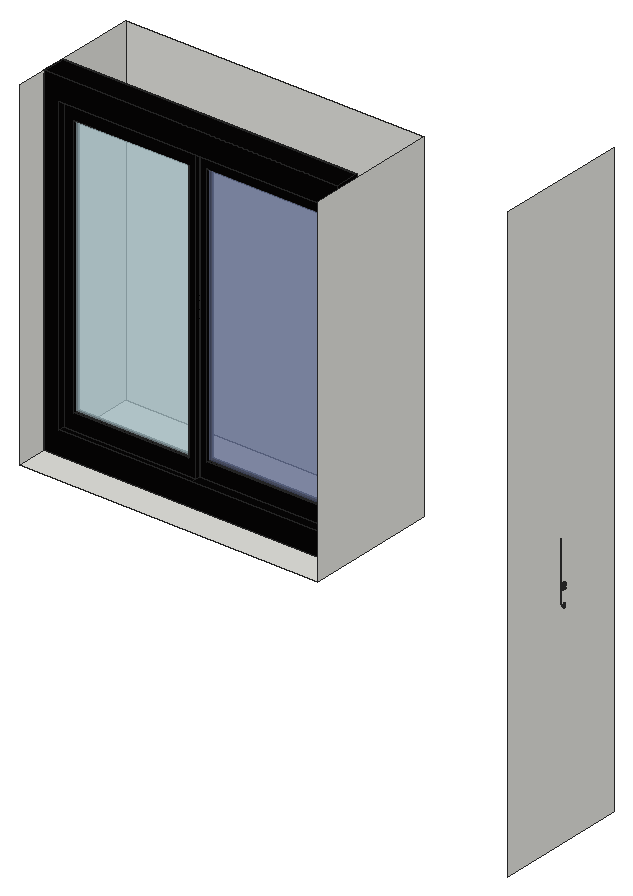
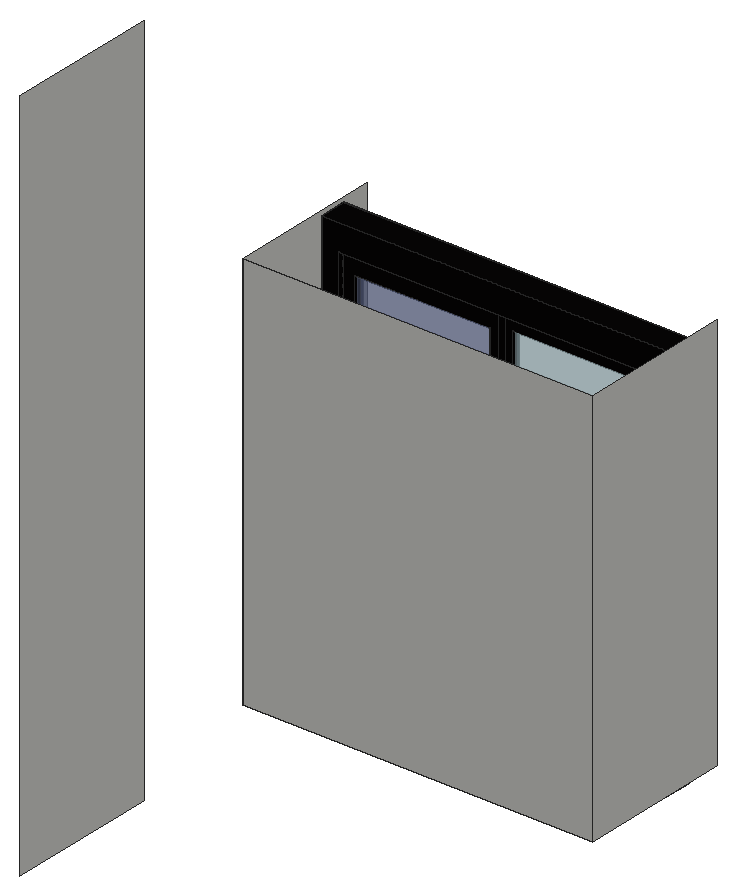
# SketchUp Ruby script. Lengths in inches.
U = 1.inch
M = Sketchup.active_model
def pt(a) = Geom::Point3d.new(a.map { |v| v * U })
def face(e, loops, mat)
  f = e.add_face(loops[0].map { |a| pt(a) })
  loops[1..].each { |l| e.add_face(l.map { |a| pt(a) }).erase! }
  f.material = f.back_material = mat if mat
  f
end
# faces: each face lists its corners as indices into pts; further lists are holes
def faces(e, pts, list, mat = nil) = list.each { |f| face(e, (f[0].is_a?(Array) ? f : [f]).map { |l| l.map { |i| pts[i] } }, mat) }
# xy, xz, yz: faces in a plane at the given z, y or x. An outline is a flat list of corners, or four numbers for a rectangle; further outlines are holes
def ring(l) = l.size == 4 ? [[l[0], l[1]], [l[2], l[1]], [l[2], l[3]], [l[0], l[3]]] : l.each_slice(2).to_a
def flat(e, list, mat, &to3) = list.each { |f| face(e, (f[0].is_a?(Array) ? f : [f]).map { |l| ring(l).map { |u, v| to3.(u, v) } }, mat) }
def xy(e, z, list, mat = nil) = flat(e, list, mat) { |x, y| [x, y, z] }
def xz(e, y, list, mat = nil) = flat(e, list, mat) { |x, z| [x, y, z] }
def yz(e, x, list, mat = nil) = flat(e, list, mat) { |y, z| [x, y, z] }
def lines(e, pts, list) = list.each { |a, b| e.add_line(pt(pts[a]), pt(pts[b])) }
# prism: a flat outline (further loops are holes) pulled along v
def prism(e, loops, v, mat = nil)
  f = face(e, loops, mat); d = Geom::Vector3d.new(v.map { |x| x * U })
  f.pushpull(f.normal.samedirection?(d) ? d.length : -d.length)
end
def box(e, o, s, mat = nil) = prism(e, [[o, [o[0] + s[0], o[1], o[2]], [o[0] + s[0], o[1] + s[1], o[2]], [o[0], o[1] + s[1], o[2]]]], [0, 0, s[2]], mat)
def at(x, y, z, deg = 0) = Geom::Transformation.translation(pt([x, y, z])) * Geom::Transformation.rotation(ORIGIN, Z_AXIS, deg.degrees)
def axes(o, x, y, z) = Geom::Transformation.new([*x, 0, *y, 0, *z, 0, *pt(o).to_a, 1])
def part(name) = M.definitions.add(name)
# library, detail: a bought-in or finely detailed component or shape, given as its bounding box
def library(name, o, s) = part(name).tap { |d| box(d.entities, o, s) }
def detail(e, o, s) = box(e.add_group.entities, o, s)
def put(e, d, t, mat = nil) = e.add_instance(d, t).tap { |i| i.material = mat if mat }
def group(e, t, mat = nil) = e.add_group.tap { |g| g.transformation = t; g.material = mat if mat }.entities
root = M.entities
M.materials.add("Generic\#5").color = [7, 6, 6]
M.materials.add("Material \#1").color = [140, 140, 140]
M.materials.add("[Translucent_Glass_Safety]").color = [204, 235, 244]
M.materials["[Translucent_Glass_Safety]"].alpha = 0.5
M.materials.add("[Translucent_Glass_Sky_Reflection]").color = [125, 138, 183]
M.materials["[Translucent_Glass_Sky_Reflection]"].alpha = 0.52
c1 = part("Sliding window")
xy(c1.entities,0,[[0,0,4.33,55.51]])
xy(c1.entities,2.76,[[0,2.76,2,27.76],[3.15,2.76,4.33,27.76],[0,27.76,0.82,52.76],[0.82,27.76,2.36,52.76],[2.36,27.76,4.33,52.76]])
xy(c1.entities,4.72,[[2,4.72,2.4,26.38],[2.76,4.72,3.15,26.38],[0.82,29.13,1.22,50.79],[1.97,29.13,2.36,50.79]])
xy(c1.entities,36.61,[[2,4.72,2.4,26.38],[2.76,4.72,3.15,26.38],[0.82,29.13,1.22,50.79],[1.97,29.13,2.36,50.79]])
xy(c1.entities,38.58,[[0,2.76,2,27.76],[3.15,2.76,4.33,27.76],[0,27.76,0.82,52.76],[0.82,27.76,2.36,52.76],[2.36,27.76,4.33,52.76]])
xy(c1.entities,41.34,[[0,0,4.33,55.51]])
xz(c1.entities,0,[[0,0,4.33,41.34]])
xz(c1.entities,2.76,[[0,2.76,2,38.58],[3.15,2.76,4.33,38.58]])
xz(c1.entities,4.72,[[2,4.72,2.4,36.61],[2.76,4.72,3.15,36.61]])
xz(c1.entities,26.38,[[2,4.72,2.4,36.61],[2.76,4.72,3.15,36.61]])
xz(c1.entities,27.76,[[0.82,2.76,2,38.58],[2,2.76,2.36,38.58],[2.36,2.76,3.15,38.58]])
xz(c1.entities,29.13,[[0.82,4.72,1.22,36.61],[1.97,4.72,2.36,36.61]])
xz(c1.entities,50.79,[[0.82,4.72,1.22,36.61],[1.97,4.72,2.36,36.61]])
xz(c1.entities,52.76,[[0,2.76,0.82,38.58],[0.82,2.76,2.36,38.58],[2.36,2.76,4.33,38.58]])
xz(c1.entities,55.51,[[0,0,4.33,41.34]])
yz(c1.entities,0,[[[0,0,55.51,41.34],[2.76,2.76,52.76,38.58]]])
yz(c1.entities,0.82,[[[27.76,2.76,52.76,38.58],[29.13,4.72,50.79,36.61]]])
yz(c1.entities,1.22,[[29.13,4.72,50.79,36.61]],"[Translucent_Glass_Sky_Reflection]")
yz(c1.entities,1.97,[[29.13,4.72,50.79,36.61]],"[Translucent_Glass_Sky_Reflection]")
yz(c1.entities,2,[[[2.76,2.76,27.76,38.58],[4.72,4.72,26.38,36.61]]])
yz(c1.entities,2.36,[[[27.76,2.76,52.76,38.58],[29.13,4.72,50.79,36.61]]])
yz(c1.entities,2.4,[[4.72,4.72,26.38,36.61]],"[Translucent_Glass_Safety]")
yz(c1.entities,2.76,[[4.72,4.72,26.38,36.61]],"[Translucent_Glass_Safety]")
yz(c1.entities,3.15,[[[2.76,2.76,27.76,38.58],[4.72,4.72,26.38,36.61]]])
yz(c1.entities,4.33,[[[0,0,55.51,41.34],[2.76,2.76,52.76,38.58]]])
xy(root,184.097,[[27.868,114.716,69.368,133.091]])
xy(root,193.609,[[101.384,117.386,101.384,117.671,101.412,117.386],[101.412,117.386,101.384,117.671,101.412,117.671]],"Material \#1")
xy(root,193.919,[[101.369,117.386,101.417,117.671,101.369,117.671]],"Material \#1")
xz(root,117.355,[[101.393,193.094,101.338,193.109,101.448,193.109],[101.393,193.094,101.364,193.098,101.338,193.109],[101.338,193.109,101.268,193.523,101.514,193.207],[101.338,193.109,101.271,193.207,101.268,193.523],[101.338,193.109,101.295,193.149,101.271,193.207],
  [101.338,193.109,101.315,193.126,101.295,193.149],[101.295,193.149,101.281,193.177,101.271,193.207],[101.514,193.207,101.265,193.54,101.263,193.545],[101.514,193.207,101.267,193.534,101.265,193.54],[101.514,193.207,101.268,193.529,101.267,193.534],
  [101.271,193.207,101.268,193.241,101.268,193.523],[101.514,193.207,101.268,193.523,101.268,193.529],[101.517,193.241,101.239,193.619,101.27,193.583],[101.517,193.241,101.263,193.545,101.239,193.619],[101.517,193.241,101.27,193.583,101.306,193.555],
  [101.517,193.241,101.306,193.555,101.348,193.538],[101.263,193.545,101.172,193.729,101.216,193.662],[101.263,193.545,101.26,193.55,101.172,193.729],[101.263,193.545,101.216,193.662,101.239,193.619],[101.26,193.55,101.257,193.555,101.172,193.729],
  [101.257,193.555,101.214,193.607,101.172,193.729],[101.257,193.555,101.253,193.559,101.214,193.607],[101.253,193.559,101.232,193.582,101.214,193.607],[101.214,193.607,101.186,193.664,101.172,193.729],[101.214,193.607,101.199,193.634,101.186,193.664],
  [101.216,193.662,101.172,193.729,101.201,193.711],[101.186,193.664,101.177,193.696,101.172,193.729],[101.201,193.711,101.172,193.729,101.196,193.764],[101.172,193.729,101.201,193.817,101.196,193.764],[101.219,193.929,101.306,193.973,101.27,193.945]],"Material \#1")
xz(root,117.386,[[101.384,193.609,101.403,193.632,101.374,193.632],[101.384,193.609,101.412,193.609,101.403,193.632],[101.374,193.632,101.408,193.64,101.369,193.64],[101.374,193.632,101.403,193.632,101.408,193.64],[101.369,193.64,101.408,193.64,101.408,193.657],
  [101.369,193.64,101.408,193.657,101.369,193.657],[101.369,193.657,101.403,193.665,101.374,193.665],[101.369,193.657,101.408,193.657,101.403,193.665],[101.374,193.665,101.403,193.665,101.412,193.694],[101.374,193.665,101.412,193.694,101.374,193.694],
  [101.374,193.694,101.412,193.694,101.412,193.721],[101.374,193.694,101.412,193.721,101.374,193.721],[101.374,193.721,101.419,193.743,101.367,193.743],[101.374,193.721,101.412,193.721,101.419,193.743],[101.367,193.743,101.419,193.743,101.419,193.765],
  [101.367,193.743,101.419,193.765,101.367,193.765],[101.367,193.765,101.412,193.787,101.374,193.787],[101.367,193.765,101.419,193.765,101.412,193.787],[101.374,193.787,101.417,193.803,101.369,193.803],[101.374,193.787,101.412,193.787,101.417,193.803],
  [101.369,193.803,101.417,193.803,101.417,193.853],[101.369,193.803,101.417,193.853,101.369,193.853],[101.369,193.853,101.411,193.857,101.375,193.857],[101.369,193.853,101.417,193.853,101.411,193.857],[101.375,193.857,101.411,193.857,101.411,193.865],
  [101.375,193.857,101.411,193.865,101.375,193.865],[101.375,193.865,101.417,193.869,101.369,193.869],[101.375,193.865,101.411,193.865,101.417,193.869],[101.369,193.869,101.417,193.869,101.417,193.919],[101.369,193.869,101.417,193.919,101.369,193.919]],"Material \#1")
xz(root,117.601,[[101.393,193.532,101.393,193.539,101.342,193.54],[101.393,193.532,101.442,193.547,101.393,193.539],[101.393,193.532,101.444,193.54,101.442,193.547],[101.393,193.539,101.344,193.547,101.342,193.54],[101.342,193.54,101.344,193.547,101.294,193.563],
  [101.444,193.54,101.488,193.57,101.442,193.547],[101.444,193.54,101.491,193.563,101.488,193.57],[101.344,193.547,101.298,193.57,101.294,193.563],[101.294,193.563,101.298,193.57,101.254,193.6],[101.491,193.563,101.527,193.605,101.488,193.57],
  [101.491,193.563,101.532,193.6,101.527,193.605],[101.298,193.57,101.258,193.605,101.254,193.6],[101.254,193.6,101.258,193.605,101.222,193.648],[101.532,193.6,101.558,193.652,101.527,193.605],[101.532,193.6,101.563,193.648,101.558,193.652],
  [101.258,193.605,101.228,193.652,101.222,193.648],[101.222,193.648,101.228,193.652,101.203,193.704],[101.563,193.648,101.577,193.706,101.558,193.652],[101.563,193.648,101.583,193.704,101.577,193.706],[101.228,193.652,101.209,193.706,101.203,193.704],
  [101.203,193.704,101.209,193.706,101.196,193.764],[101.583,193.704,101.583,193.764,101.577,193.706],[101.583,193.704,101.59,193.764,101.583,193.764],[101.209,193.706,101.203,193.764,101.196,193.764],[101.196,193.764,101.203,193.764,101.203,193.824],
  [101.203,193.764,101.209,193.822,101.203,193.824],[101.583,193.764,101.59,193.764,101.577,193.822],[101.59,193.764,101.583,193.824,101.577,193.822],[101.209,193.822,101.222,193.88,101.203,193.824],[101.209,193.822,101.228,193.876,101.222,193.88],
  [101.577,193.822,101.583,193.824,101.558,193.876],[101.583,193.824,101.563,193.88,101.558,193.876],[101.228,193.876,101.254,193.928,101.222,193.88],[101.228,193.876,101.258,193.923,101.254,193.928],[101.558,193.876,101.563,193.88,101.527,193.923],
  [101.563,193.88,101.532,193.928,101.527,193.923],[101.258,193.923,101.294,193.965,101.254,193.928],[101.258,193.923,101.298,193.958,101.294,193.965],[101.527,193.923,101.532,193.928,101.488,193.958],[101.532,193.928,101.491,193.965,101.488,193.958],
  [101.298,193.958,101.342,193.988,101.294,193.965],[101.298,193.958,101.344,193.981,101.342,193.988],[101.488,193.958,101.491,193.965,101.442,193.981],[101.491,193.965,101.444,193.988,101.442,193.981],[101.344,193.981,101.393,193.996,101.342,193.988],
  [101.344,193.981,101.393,193.989,101.393,193.996],[101.442,193.981,101.444,193.988,101.393,193.989],[101.444,193.988,101.393,193.996,101.393,193.989]],"Material \#1")
xz(root,117.632,[[101.393,190.763,101.393,190.775,101.29,190.774],[101.29,190.774,101.291,190.785,101.193,190.805],[101.29,190.774,101.393,190.775,101.291,190.785],[101.291,190.785,101.196,190.816,101.193,190.805],[101.193,190.805,101.196,190.816,101.103,190.856],
  [101.196,190.816,101.108,190.866,101.103,190.856],[101.103,190.856,101.108,190.866,101.023,190.922],[101.108,190.866,101.03,190.931,101.023,190.922],[101.023,190.922,101.03,190.931,100.954,191.004],[101.03,190.931,100.961,191.012,100.954,191.004],
  [101.393,190.944,101.393,190.956,101.359,190.948],[101.359,190.948,101.36,190.959,101.326,190.958],[101.359,190.948,101.393,190.956,101.36,190.959],[101.326,190.958,101.33,190.969,101.297,190.975],[101.326,190.958,101.36,190.959,101.33,190.969],
  [101.33,190.969,101.302,190.985,101.297,190.975],[101.297,190.975,101.302,190.985,101.27,190.997],[101.302,190.985,101.276,191.006,101.27,190.997],[101.27,190.997,101.276,191.006,101.247,191.024],[100.954,191.004,100.961,191.012,100.9,191.093],
  [101.276,191.006,101.255,191.032,101.247,191.024],[100.961,191.012,100.909,191.099,100.9,191.093],[101.247,191.024,101.255,191.032,101.228,191.056],[101.255,191.032,101.237,191.062,101.228,191.056],[101.228,191.056,101.237,191.062,101.214,191.091],
  [101.237,191.062,101.223,191.095,101.214,191.091],[101.214,191.091,101.223,191.095,101.205,191.129],[100.9,191.093,100.909,191.099,100.855,191.204],[101.223,191.095,101.215,191.131,101.205,191.129],[100.909,191.099,100.864,191.208,100.855,191.204],
  [101.205,191.129,101.215,191.131,101.202,191.165],[101.215,191.131,101.212,191.165,101.202,191.165],[101.202,191.165,101.212,191.165,101.205,191.21],[101.212,191.165,101.215,191.207,101.205,191.21],[100.855,191.204,100.864,191.208,100.828,191.319],
  [101.215,191.207,101.214,191.248,101.205,191.21],[101.215,191.207,101.223,191.244,101.214,191.248],[100.864,191.208,100.838,191.321,100.828,191.319],[101.223,191.244,101.228,191.283,101.214,191.248],[101.223,191.244,101.237,191.277,101.228,191.283],
  [101.237,191.277,101.247,191.314,101.228,191.283],[101.237,191.277,101.255,191.307,101.247,191.314],[101.255,191.307,101.27,191.341,101.247,191.314],[101.255,191.307,101.276,191.332,101.27,191.341],[100.828,191.319,100.838,191.321,100.819,191.445],
  [100.838,191.321,100.828,191.445,100.819,191.445],[101.276,191.332,101.297,191.364,101.27,191.341],[101.276,191.332,101.302,191.353,101.297,191.364],[101.302,191.353,101.326,191.38,101.297,191.364],[101.302,191.353,101.33,191.369,101.326,191.38],
  [101.33,191.369,101.359,191.391,101.326,191.38],[101.33,191.369,101.36,191.379,101.359,191.391],[101.36,191.379,101.393,191.394,101.359,191.391],[101.36,191.379,101.393,191.383,101.393,191.394],[100.819,191.445,100.828,191.445,100.819,199.181],
  [100.828,191.445,100.828,199.181,100.819,199.181]],"Material \#1")
xz(root,117.662,[[101.393,193.094,101.295,193.149,101.338,193.109],[101.393,193.094,101.49,193.149,101.295,193.149],[101.393,193.094,101.338,193.109,101.364,193.098],[101.338,193.109,101.295,193.149,101.315,193.126],[101.49,193.149,101.172,193.729,101.263,193.545],
  [101.49,193.149,101.239,193.619,101.172,193.729],[101.49,193.149,101.27,193.583,101.239,193.619],[101.49,193.149,101.263,193.545,101.265,193.54],[101.49,193.149,101.265,193.54,101.267,193.534],[101.49,193.149,101.267,193.534,101.268,193.529],
  [101.295,193.149,101.268,193.523,101.271,193.207],[101.295,193.149,101.268,193.529,101.268,193.523],[101.295,193.149,101.49,193.149,101.268,193.529],[101.49,193.149,101.306,193.555,101.27,193.583],[101.295,193.149,101.271,193.207,101.281,193.177],
  [101.49,193.149,101.348,193.538,101.306,193.555],[101.271,193.207,101.268,193.523,101.268,193.241],[101.263,193.545,101.172,193.729,101.26,193.55],[101.26,193.55,101.172,193.729,101.257,193.555],[101.257,193.555,101.172,193.729,101.214,193.607],
  [101.257,193.555,101.214,193.607,101.253,193.559],[101.253,193.559,101.214,193.607,101.232,193.582],[101.214,193.607,101.172,193.729,101.186,193.664],[101.214,193.607,101.186,193.664,101.199,193.634],[101.239,193.619,101.216,193.662,101.172,193.729],
  [101.216,193.662,101.201,193.711,101.172,193.729],[101.186,193.664,101.172,193.729,101.177,193.696],[101.201,193.711,101.196,193.764,101.172,193.729],[101.172,193.729,101.176,193.824,101.17,193.764],[101.172,193.729,101.196,193.764,101.201,193.817],
  [101.172,193.729,101.201,193.817,101.219,193.929],[101.172,193.729,101.219,193.929,101.176,193.824],[101.201,193.817,101.216,193.866,101.219,193.929],[101.176,193.824,101.219,193.929,101.192,193.88],[101.216,193.866,101.239,193.909,101.219,193.929],
  [101.239,193.909,101.27,193.945,101.219,193.929],[101.219,193.929,101.27,193.945,101.306,193.973],[101.219,193.929,101.295,194.001,101.253,193.969],[101.219,193.929,101.306,193.973,101.393,194.027],[101.219,193.929,101.393,194.027,101.295,194.001],
  [101.306,193.973,101.348,193.99,101.393,194.027],[101.348,193.99,101.393,193.996,101.393,194.027],[101.295,194.001,101.393,194.027,101.342,194.02]],"Material \#1")
xz(root,117.671,[[101.393,193.557,101.393,193.565,101.347,193.564],[101.393,193.557,101.436,193.572,101.393,193.565],[101.393,193.557,101.438,193.564,101.436,193.572],[101.347,193.564,101.349,193.572,101.305,193.585],[101.347,193.564,101.393,193.565,101.349,193.572],
  [101.438,193.564,101.477,193.591,101.436,193.572],[101.438,193.564,101.481,193.585,101.477,193.591],[101.349,193.572,101.308,193.591,101.305,193.585],[101.305,193.585,101.308,193.591,101.269,193.618],[101.481,193.585,101.512,193.623,101.477,193.591],
  [101.481,193.585,101.517,193.618,101.512,193.623],[101.308,193.591,101.273,193.623,101.269,193.618],[101.269,193.618,101.273,193.623,101.241,193.66],[101.517,193.618,101.539,193.664,101.512,193.623],[101.517,193.618,101.545,193.66,101.539,193.664],
  [101.273,193.623,101.247,193.664,101.241,193.66],[101.241,193.66,101.247,193.664,101.223,193.71],[101.545,193.66,101.556,193.712,101.539,193.664],[101.545,193.66,101.562,193.71,101.556,193.712],[101.247,193.664,101.23,193.712,101.223,193.71],
  [101.223,193.71,101.23,193.712,101.217,193.764],[101.562,193.71,101.562,193.764,101.556,193.712],[101.562,193.71,101.568,193.764,101.562,193.764],[101.23,193.712,101.224,193.764,101.217,193.764],[101.217,193.764,101.224,193.764,101.223,193.818],
  [101.224,193.764,101.23,193.816,101.223,193.818],[101.562,193.764,101.568,193.764,101.556,193.816],[101.568,193.764,101.562,193.818,101.556,193.816],[101.23,193.816,101.241,193.868,101.223,193.818],[101.23,193.816,101.247,193.864,101.241,193.868],
  [101.556,193.816,101.562,193.818,101.539,193.864],[101.562,193.818,101.545,193.868,101.539,193.864],[101.247,193.864,101.269,193.91,101.241,193.868],[101.247,193.864,101.273,193.905,101.269,193.91],[101.539,193.864,101.545,193.868,101.512,193.905],
  [101.545,193.868,101.517,193.91,101.512,193.905],[101.273,193.905,101.305,193.943,101.269,193.91],[101.273,193.905,101.308,193.937,101.305,193.943],[101.512,193.905,101.517,193.91,101.477,193.937],[101.517,193.91,101.481,193.943,101.477,193.937],
  [101.308,193.937,101.347,193.964,101.305,193.943],[101.308,193.937,101.349,193.956,101.347,193.964],[101.477,193.937,101.481,193.943,101.436,193.956],[101.481,193.943,101.438,193.964,101.436,193.956],[101.349,193.956,101.393,193.971,101.347,193.964],
  [101.349,193.956,101.393,193.963,101.393,193.971],[101.436,193.956,101.438,193.964,101.393,193.963],[101.393,193.963,101.438,193.964,101.393,193.971]],"Material \#1")
xz(root,133.091,[[27.868,184.097,69.368,231.472]])
yz(root,27.868,[[114.716,184.097,133.091,231.472]])
yz(root,69.368,[[114.716,184.097,133.091,231.472]])
yz(root,95.815,[[114.716,156.586,133.091,239.461]])
yz(root,101.369,[[117.386,193.869,117.386,193.919,117.671,193.919]],"Material \#1")
yz(root,101.374,[[117.386,193.665,117.386,193.694,117.671,193.694]],"Material \#1")
p = [[101.329,117.625,191.062],[101.349,117.625,191.05],[101.349,117.601,191.05],[101.329,117.601,191.062],[101.363,117.632,191.074],[101.363,117.607,191.074],
  [101.409,117.634,191.243],[101.34,117.634,191.126],[101.34,117.61,191.126],[101.409,117.61,191.243],[101.327,117.632,191.104],[101.327,117.607,191.104],
  [101.3125,117.625,191.08],[101.3125,117.601,191.08],[101.376,117.634,191.096],[101.376,117.61,191.096],[101.446,117.634,191.213],[101.446,117.61,191.213],
  [101.459,117.632,191.235],[101.459,117.607,191.235],[101.422,117.632,191.265],[101.422,117.607,191.265],[101.473,117.625,191.259],[101.473,117.601,191.259],
  [101.456,117.625,191.277],[101.437,117.625,191.289],[101.437,117.601,191.289],[101.456,117.601,191.277],[101.372,117.671,193.636],[101.384,117.671,193.609],
  [101.384,117.386,193.609],[101.374,117.386,193.632],[101.372,117.671,193.636],[101.372,117.671,193.636],[101.374,117.386,193.632],[101.369,117.386,193.64],
  [101.372,117.671,193.661],[101.372,117.671,193.636],[101.369,117.386,193.64],[101.369,117.386,193.657],[101.372,117.671,193.661],[101.369,117.386,193.657],
  [101.374,117.386,193.665],[101.367,117.386,193.743],[101.367,117.386,193.765],[101.37,117.671,193.776],[101.374,117.386,193.721],[101.367,117.386,193.743],
  [101.367,117.671,193.754],[101.374,117.386,193.694],[101.374,117.386,193.721],[101.37,117.671,193.732],[101.374,117.671,193.694],[101.372,117.671,193.661],
  [101.374,117.386,193.665],[101.37,117.671,193.776],[101.367,117.671,193.754],[101.367,117.386,193.743],[101.367,117.671,193.754],[101.37,117.671,193.732],
  [101.374,117.386,193.721],[101.37,117.671,193.732],[101.374,117.671,193.694],[101.374,117.386,193.694],[101.369,117.386,193.803],[101.369,117.386,193.853],
  [101.371,117.671,193.857],[101.374,117.386,193.787],[101.369,117.386,193.803],[101.369,117.671,193.806],[101.367,117.386,193.765],[101.374,117.386,193.787],
  [101.372,117.671,193.795],[101.371,117.671,193.857],[101.369,117.671,193.806],[101.369,117.386,193.803],[101.369,117.671,193.806],[101.372,117.671,193.795],
  [101.374,117.386,193.787],[101.372,117.671,193.795],[101.37,117.671,193.776],[101.367,117.386,193.765],[101.414,117.671,193.862],[101.411,117.386,193.857],
  [101.417,117.386,193.853],[101.371,117.671,193.857],[101.375,117.386,193.857],[101.375,117.386,193.865],[101.371,117.671,193.857],[101.369,117.386,193.869],
  [101.371,117.671,193.857],[101.369,117.386,193.853],[101.414,117.671,193.862],[101.417,117.386,193.869],[101.411,117.386,193.865],[101.414,117.671,193.862],
  [101.369,117.671,193.919],[101.371,117.671,193.857],[101.369,117.386,193.869]]
faces(root,p,[[0,1,2],[2,3,0],[1,4,5],[5,2,1],[6,7,8],[8,9,6],[7,10,11],[11,8,7],
  [10,12,13],[13,11,10],[12,0,3],[3,13,12],[4,14,15],[15,5,4],[14,16,17],[17,15,14],
  [16,18,19],[19,17,16],[20,6,9],[9,21,20],[18,22,23],[23,19,18],[24,25,26],[26,27,24],
  [25,20,21],[21,26,25],[22,24,27],[27,23,22],[28,29,30],[30,31,32],[33,34,35],[36,37,38],
  [38,39,36],[40,41,42],[43,44,45],[46,47,48],[49,50,51],[52,53,54],[55,56,57],[58,59,60],
  [61,62,63],[64,65,66],[67,68,69],[70,71,72],[73,74,75],[76,77,78],[79,80,81],[82,83,84],
  [85,86,87],[88,87,89],[90,91,86],[92,93,94],[95,94,83],[96,97,98]],"Material \#1")
put(root,c1,axes([27.87,122.1,184.1],[0,-0.7372,0],[0.7372,0,0],[0,0,1.14602]),"Generic\#5")
